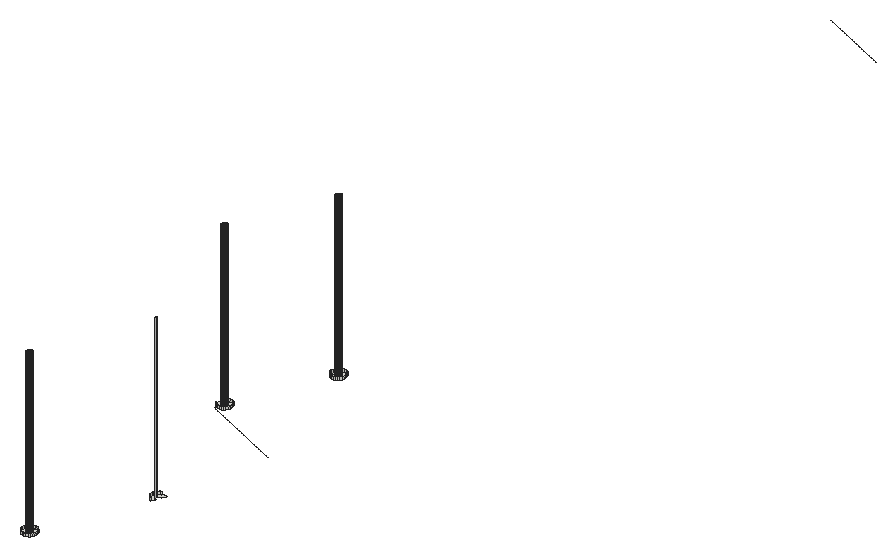
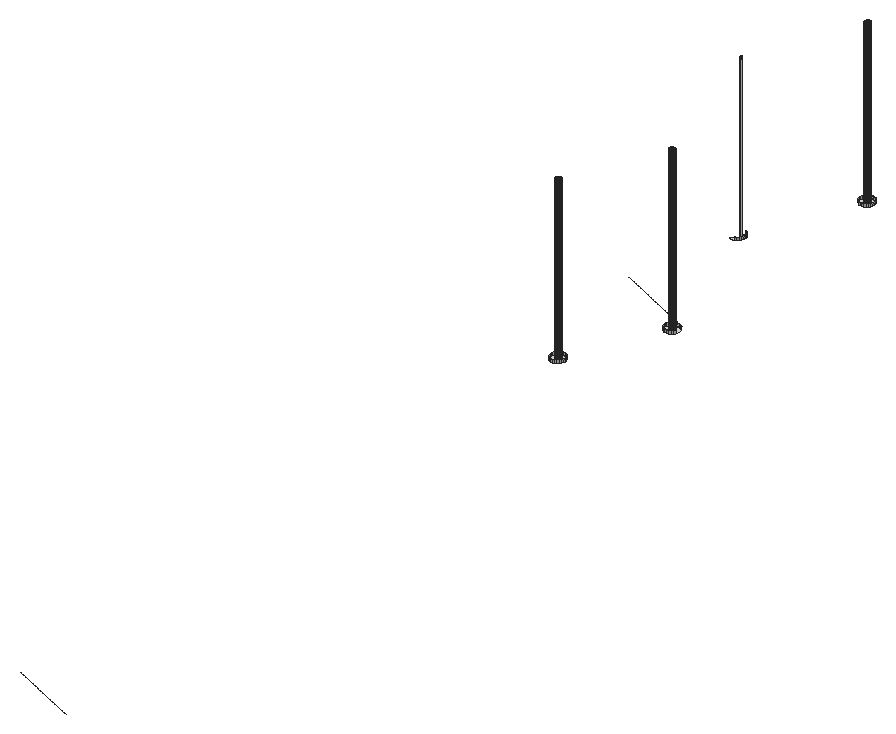
# SketchUp Ruby script. Lengths in inches.
U = 1.inch
M = Sketchup.active_model
def pt(a) = Geom::Point3d.new(a.map { |v| v * U })
def face(e, loops, mat)
  f = e.add_face(loops[0].map { |a| pt(a) })
  loops[1..].each { |l| e.add_face(l.map { |a| pt(a) }).erase! }
  f.material = f.back_material = mat if mat
  f
end
# faces: each face lists its corners as indices into pts; further lists are holes
def faces(e, pts, list, mat = nil) = list.each { |f| face(e, (f[0].is_a?(Array) ? f : [f]).map { |l| l.map { |i| pts[i] } }, mat) }
# xy, xz, yz: faces in a plane at the given z, y or x. An outline is a flat list of corners, or four numbers for a rectangle; further outlines are holes
def ring(l) = l.size == 4 ? [[l[0], l[1]], [l[2], l[1]], [l[2], l[3]], [l[0], l[3]]] : l.each_slice(2).to_a
def flat(e, list, mat, &to3) = list.each { |f| face(e, (f[0].is_a?(Array) ? f : [f]).map { |l| ring(l).map { |u, v| to3.(u, v) } }, mat) }
def xy(e, z, list, mat = nil) = flat(e, list, mat) { |x, y| [x, y, z] }
def xz(e, y, list, mat = nil) = flat(e, list, mat) { |x, z| [x, y, z] }
def yz(e, x, list, mat = nil) = flat(e, list, mat) { |y, z| [x, y, z] }
def lines(e, pts, list) = list.each { |a, b| e.add_line(pt(pts[a]), pt(pts[b])) }
# prism: a flat outline (further loops are holes) pulled along v
def prism(e, loops, v, mat = nil)
  f = face(e, loops, mat); d = Geom::Vector3d.new(v.map { |x| x * U })
  f.pushpull(f.normal.samedirection?(d) ? d.length : -d.length)
end
def box(e, o, s, mat = nil) = prism(e, [[o, [o[0] + s[0], o[1], o[2]], [o[0] + s[0], o[1] + s[1], o[2]], [o[0], o[1] + s[1], o[2]]]], [0, 0, s[2]], mat)
def at(x, y, z, deg = 0) = Geom::Transformation.translation(pt([x, y, z])) * Geom::Transformation.rotation(ORIGIN, Z_AXIS, deg.degrees)
def axes(o, x, y, z) = Geom::Transformation.new([*x, 0, *y, 0, *z, 0, *pt(o).to_a, 1])
def part(name) = M.definitions.add(name)
# library, detail: a bought-in or finely detailed component or shape, given as its bounding box
def library(name, o, s) = part(name).tap { |d| box(d.entities, o, s) }
def detail(e, o, s) = box(e.add_group.entities, o, s)
def put(e, d, t, mat = nil) = e.add_instance(d, t).tap { |i| i.material = mat if mat }
def group(e, t, mat = nil) = e.add_group.tap { |g| g.transformation = t; g.material = mat if mat }.entities
root = M.entities
M.materials.add("[Color_000]").color = [255, 255, 255]
xy(root,321.27,[[[963.53,810.32,963.9375,810.4,964.3,810.59,964.61,810.86,964.84,811.2,964.97,811.59,964.99,812,964.91,812.4,964.73,812.77,964.45,813.08,964.11,813.31,964.05,813.33,963.72,813.4375,963.31,813.46,962.91,813.38,962.54,813.19,962.23,812.92,962.01,812.58,961.875,812.1875,961.85,811.78,961.93,811.375,962.12,811.01,962.39,810.7,962.73,810.47,962.8,810.45,963.125,810.34],[963.47,811.26,963.3,811.27,963.17,811.3125,963.15,811.32,963.01,811.41,962.9,811.54,962.83,811.68,962.79,811.84,962.8,812.01,962.86,812.16,962.95,812.3,963.07,812.41,963.22,812.48,963.375,812.52,963.54,812.51,963.67,812.46,963.7,812.46,963.83,812.37,963.94,812.24,964.02,812.1,964.05,811.93,964.04,811.77,963.99,811.61,963.9,811.48,963.77,811.37,963.63,811.29]],[962.8,810.45,963.17,811.3125,963.15,811.32,963.01,811.41,962.9,811.54,962.83,811.68,962.79,811.84,962.8,812.01,962.86,812.16,962.95,812.3,963.07,812.41,963.22,812.48,963.375,812.52,963.54,812.51,963.67,812.46,964.05,813.33,963.72,813.4375,963.31,813.46,962.91,813.38,962.54,813.19,962.23,812.92,962.01,812.58,961.875,812.1875,961.85,811.78,961.93,811.375,962.12,811.01,962.39,810.7,962.73,810.47],[963.17,811.3125,963.67,812.46,963.54,812.51,963.375,812.52,963.22,812.48,963.07,812.41,962.95,812.3,962.86,812.16,962.8,812.01,962.79,811.84,962.83,811.68,962.9,811.54,963.01,811.41,963.15,811.32],[972.96,833.79,973.34,834.66,973.3125,834.66,973.18,834.75,973.07,834.88,972.99,835.02,972.96,835.1875,972.97,835.35,973.02,835.51,973.11,835.64,973.23,835.75,973.38,835.83,973.54,835.86,973.71,835.85,973.84,835.81,974.21,836.67,973.89,836.78,973.48,836.8,973.07,836.72,972.7,836.53,972.4,836.26,972.17,835.92,972.04,835.53,972.02,835.12,972.1,834.72,972.28,834.35,972.56,834.04,972.9,833.8125],[[961.92,866.71,962.32,866.79,962.6875,866.97,962.99,867.25,963.22,867.59,963.35,867.98,963.375,868.39,963.29,868.79,963.11,869.16,962.83,869.47,962.49,869.69,962.43,869.72,962.1,869.82,961.69,869.85,961.29,869.77,960.92,869.58,960.61,869.31,960.39,868.97,960.26,868.58,960.23,868.17,960.32,867.76,960.5,867.4,960.77,867.09,961.12,866.86,961.51,866.73],[961.85,867.65,961.68,867.66,961.55,867.7,961.53,867.71,961.39,867.8,961.28,867.93,961.21,868.07,961.18,868.23,961.18,868.4,961.24,868.55,961.33,868.69,961.45,868.8,961.6,868.875,961.76,868.91,961.92,868.9,962.05,868.85,962.08,868.84,962.22,868.75,962.32,868.63,962.4,868.48,962.43,868.32,962.42,868.16,962.37,868,962.28,867.87,962.16,867.76,962.01,867.68]],
  [961.18,866.84,961.55,867.7,961.53,867.71,961.39,867.8,961.28,867.93,961.21,868.07,961.18,868.23,961.18,868.4,961.24,868.55,961.33,868.69,961.45,868.8,961.6,868.875,961.76,868.91,961.92,868.9,962.05,868.85,962.43,869.72,962.1,869.82,961.69,869.85,961.29,869.77,960.92,869.58,960.61,869.31,960.39,868.97,960.26,868.58,960.23,868.17,960.32,867.76,960.5,867.4,960.77,867.09,961.12,866.86],[961.55,867.7,962.05,868.85,961.92,868.9,961.76,868.91,961.6,868.875,961.45,868.8,961.33,868.69,961.24,868.55,961.18,868.4,961.18,868.23,961.21,868.07,961.28,867.93,961.39,867.8,961.53,867.71],[[970.875,887.27,971.28,887.36,971.64,887.54,971.95,887.8125,972.18,888.16,972.31,888.55,972.33,888.96,972.25,889.36,972.06,889.73,971.79,890.04,971.45,890.26,971.06,890.39,970.65,890.42,970.25,890.33,969.88,890.15,969.57,889.875,969.34,889.53,969.21,889.14,969.19,888.73,969.27,888.33,969.46,887.96,969.73,887.65,970.07,887.43,970.46,887.3],[970.81,888.22,970.64,888.23,970.51,888.27,970.49,888.28,970.35,888.37,970.24,888.49,970.17,888.64,970.13,888.8,970.14,888.96,970.19,889.12,970.28,889.26,970.41,889.37,970.55,889.44,970.72,889.47,970.88,889.46,971.01,889.42,971.04,889.41,971.17,889.32,971.28,889.2,971.36,889.05,971.39,888.89,971.38,888.73,971.33,888.57,971.24,888.43,971.11,888.32,970.97,888.25]],[970.13,887.41,970.51,888.27,970.49,888.28,970.35,888.37,970.24,888.49,970.17,888.64,970.13,888.8,970.14,888.96,970.19,889.12,970.28,889.26,970.41,889.37,970.55,889.44,970.72,889.47,970.88,889.46,971.01,889.42,971.39,890.28,971.06,890.39,970.65,890.42,970.25,890.33,969.88,890.15,969.57,889.875,969.34,889.53,969.21,889.14,969.19,888.73,969.27,888.33,969.46,887.96,969.73,887.65,970.07,887.43],[970.51,888.27,971.01,889.42,970.88,889.46,970.72,889.47,970.55,889.44,970.41,889.37,970.28,889.26,970.19,889.12,970.14,888.96,970.13,888.8,970.17,888.64,970.24,888.49,970.35,888.37,970.49,888.28]])
xy(root,321.27,[[963.47,811.26,963.63,811.29,963.77,811.37,963.9,811.48,963.99,811.61,964.04,811.77,964.05,811.93,964.02,812.1,963.94,812.24,963.83,812.37,963.7,812.46,963.67,812.46,963.17,811.3125,963.3,811.27],[961.85,867.65,962.01,867.68,962.16,867.76,962.28,867.87,962.37,868,962.42,868.16,962.43,868.32,962.4,868.48,962.32,868.63,962.22,868.75,962.08,868.84,962.05,868.85,961.55,867.7,961.68,867.66],[970.81,888.22,970.97,888.25,971.11,888.32,971.24,888.43,971.33,888.57,971.38,888.73,971.39,888.89,971.36,889.05,971.28,889.2,971.17,889.32,971.04,889.41,971.01,889.42,970.51,888.27,970.64,888.23]],"[Color_000]")
yz(root,961.18,[[868.23,321.27,868.4,357.27]],"[Color_000]")
p = [[962.73,810.47,321.27],[962.8,810.45,321.27],[963.125,810.34,321.27],[963.125,810.34,321.86],[962.73,810.47,321.86],[963.53,810.32,321.27],
  [963.53,810.32,321.86],[963.9375,810.4,321.27],[963.9375,810.4,321.86],[964.3,810.59,321.27],[964.3,810.59,321.86],[962.39,810.7,321.27],
  [962.39,810.7,321.86],[964.61,810.86,321.27],[964.61,810.86,321.86],[962.12,811.01,321.27],[962.12,811.01,321.86],[964.84,811.2,321.27],
  [964.84,811.2,321.86],[961.93,811.375,321.27],[961.93,811.375,321.86],[964.97,811.59,321.27],[964.97,811.59,321.86],[963.01,811.41,321.27],
  [963.15,811.32,321.27],[963.15,811.32,357.27],[963.01,811.41,357.27],[963.17,811.3125,321.27],[963.3,811.27,321.27],[963.3,811.27,357.27],
  [963.47,811.26,321.27],[963.47,811.26,357.27],[963.63,811.29,321.27],[963.63,811.29,357.27],[963.77,811.37,321.27],[963.77,811.37,357.27],
  [961.85,811.78,321.27],[961.85,811.78,321.86],[962.9,811.54,321.27],[962.9,811.54,357.27],[963.9,811.48,321.27],[963.9,811.48,357.27],
  [962.83,811.68,321.27],[962.83,811.68,357.27],[963.99,811.61,321.27],[963.99,811.61,357.27],[964.04,811.77,321.27],[964.04,811.77,357.27],
  [964.99,812,321.27],[964.99,812,321.86],[962.79,811.84,321.27],[962.79,811.84,357.27],[961.875,812.1875,321.27],[961.875,812.1875,321.86],
  [962.8,812.01,321.27],[962.8,812.01,357.27],[964.05,811.93,321.27],[964.05,811.93,357.27],[964.02,812.1,321.27],[964.02,812.1,357.27],
  [962.86,812.16,321.27],[962.86,812.16,357.27],[964.91,812.4,321.27],[964.91,812.4,321.86],[963.94,812.24,321.27],[963.94,812.24,357.27],
  [962.01,812.58,321.27],[962.01,812.58,321.86],[962.95,812.3,321.27],[962.95,812.3,357.27],[963.83,812.37,321.27],[963.83,812.37,357.27],
  [963.07,812.41,321.27],[963.07,812.41,357.27],[963.22,812.48,321.27],[963.22,812.48,357.27],[963.7,812.46,321.27],[963.7,812.46,357.27],
  [964.73,812.77,321.27],[964.73,812.77,321.86],[963.375,812.52,321.27],[963.375,812.52,357.27],[963.54,812.51,321.27],[963.54,812.51,357.27],
  [963.67,812.46,321.27],[962.23,812.92,321.27],[962.23,812.92,321.86],[964.45,813.08,321.27],[964.45,813.08,321.86],[962.54,813.19,321.27],
  [962.54,813.19,321.86],[964.11,813.31,321.27],[964.11,813.31,321.86],[962.91,813.38,321.27],[962.91,813.38,321.86],[964.05,813.33,321.27],
  [963.72,813.4375,321.27],[963.72,813.4375,321.86],[963.31,813.46,321.27],[963.31,813.46,321.86],[972.56,834.04,321.27],[972.9,833.8125,321.27],
  [972.9,833.8125,321.86],[972.56,834.04,321.86],[972.28,834.35,321.27],[972.28,834.35,321.86],[972.1,834.72,321.27],[972.1,834.72,321.86],
  [972.02,835.12,321.27],[972.02,835.12,321.86],[972.99,835.02,321.27],[973.07,834.88,321.27],[973.07,834.88,357.27],[972.99,835.02,357.27],
  [972.96,835.1875,321.27],[972.96,835.1875,357.27],[972.04,835.53,321.27],[972.04,835.53,321.86],[972.97,835.35,321.27],[972.97,835.35,357.27],
  [973.02,835.51,321.27],[973.02,835.51,357.27],[972.17,835.92,321.27],[972.17,835.92,321.86],[972.4,836.26,321.27],[972.4,836.26,321.86],
  [972.7,836.53,321.27],[972.7,836.53,321.86],[973.07,836.72,321.27],[973.07,836.72,321.86],[961.12,866.86,321.27],[961.18,866.84,321.27],
  [961.51,866.73,321.27],[961.51,866.73,321.86],[961.12,866.86,321.86],[961.92,866.71,321.27],[961.92,866.71,321.86],[962.32,866.79,321.27],
  [962.32,866.79,321.86],[962.6875,866.97,321.27],[962.6875,866.97,321.86],[960.77,867.09,321.27],[960.77,867.09,321.86],[962.99,867.25,321.27],
  [962.99,867.25,321.86],[960.5,867.4,321.27],[960.5,867.4,321.86],[963.22,867.59,321.27],[963.22,867.59,321.86],[961.68,867.66,321.27],
  [961.85,867.65,321.27],[961.85,867.65,357.27],[961.68,867.66,357.27],[962.01,867.68,321.27],[962.01,867.68,357.27],[963.35,867.98,321.27],
  [963.35,867.98,321.86],[961.39,867.8,321.27],[961.53,867.71,321.27],[961.53,867.71,357.27],[961.39,867.8,357.27],[961.55,867.7,321.27],
  [962.16,867.76,321.27],[962.16,867.76,357.27],[961.28,867.93,321.27],[961.28,867.93,357.27],[962.28,867.87,321.27],[962.28,867.87,357.27],
  [961.21,868.07,321.27],[961.21,868.07,357.27],[962.37,868,321.27],[962.37,868,357.27],[962.42,868.16,321.27],[962.42,868.16,357.27],
  [963.375,868.39,321.27],[963.375,868.39,321.86],[961.18,868.23,321.27],[961.18,868.23,357.27],[962.43,868.32,321.27],[962.43,868.32,357.27],
  [962.4,868.48,321.27],[962.4,868.48,357.27],[961.24,868.55,321.27],[961.18,868.4,321.27],[961.18,868.4,357.27],[961.24,868.55,357.27],
  [963.29,868.79,321.27],[963.29,868.79,321.86],[962.32,868.63,321.27],[962.32,868.63,357.27],[961.33,868.69,321.27],[961.33,868.69,357.27],
  [962.22,868.75,321.27],[962.22,868.75,357.27],[961.45,868.8,321.27],[961.45,868.8,357.27],[961.6,868.875,321.27],[961.6,868.875,357.27],
  [962.08,868.84,321.27],[962.05,868.85,321.27],[961.92,868.9,321.27],[961.92,868.9,357.27],[962.08,868.84,357.27],[963.11,869.16,321.27],
  [963.11,869.16,321.86],[961.76,868.91,321.27],[961.76,868.91,357.27],[960.61,869.31,321.27],[960.39,868.97,321.27],[960.39,868.97,321.86],
  [960.61,869.31,321.86],[962.83,869.47,321.27],[962.83,869.47,321.86],[960.92,869.58,321.27],[960.92,869.58,321.86],[962.49,869.69,321.27],
  [962.49,869.69,321.86],[961.29,869.77,321.27],[961.29,869.77,321.86],[962.43,869.72,321.27],[962.1,869.82,321.27],[962.1,869.82,321.86],
  [961.69,869.85,321.27],[961.69,869.85,321.86],[970.07,887.43,321.27],[970.13,887.41,321.27],[970.46,887.3,321.27],[970.46,887.3,321.86],
  [970.07,887.43,321.86],[970.875,887.27,321.27],[970.875,887.27,321.86],[971.28,887.36,321.27],[971.28,887.36,321.86],[969.73,887.65,321.27],
  [969.73,887.65,321.86],[971.64,887.54,321.27],[971.64,887.54,321.86],[971.95,887.8125,321.27],[971.95,887.8125,321.86],[969.46,887.96,321.27],
  [969.46,887.96,321.86],[972.18,888.16,321.27],[972.18,888.16,321.86],[969.27,888.33,321.27],[969.27,888.33,321.86],[970.49,888.28,321.27],
  [970.51,888.27,321.27],[970.64,888.23,321.27],[970.64,888.23,357.27],[970.49,888.28,357.27],[970.81,888.22,321.27],[970.81,888.22,357.27],
  [970.97,888.25,321.27],[970.97,888.25,357.27],[971.11,888.32,321.27],[971.11,888.32,357.27],[972.31,888.55,321.27],[972.31,888.55,321.86],
  [969.19,888.73,321.27],[969.19,888.73,321.86],[970.35,888.37,321.27],[970.35,888.37,357.27],[971.24,888.43,321.27],[971.24,888.43,357.27],
  [970.24,888.49,321.27],[970.24,888.49,357.27],[971.33,888.57,321.27],[971.33,888.57,357.27],[970.17,888.64,321.27],[970.17,888.64,357.27],
  [972.33,888.96,321.27],[972.33,888.96,321.86],[970.13,888.8,321.27],[970.13,888.8,357.27],[971.38,888.73,321.27],[971.38,888.73,357.27],
  [969.21,889.14,321.27],[969.21,889.14,321.86],[971.39,888.89,321.27],[971.39,888.89,357.27],[970.14,888.96,321.27],[970.14,888.96,357.27],
  [971.36,889.05,321.27],[971.36,889.05,357.27],[970.19,889.12,321.27],[970.19,889.12,357.27],[972.25,889.36,321.27],[972.25,889.36,321.86],
  [969.34,889.53,321.27],[969.34,889.53,321.86],[970.28,889.26,321.27],[970.28,889.26,357.27],[971.28,889.2,321.27],[971.28,889.2,357.27],
  [971.17,889.32,321.27],[971.17,889.32,357.27],[970.41,889.37,321.27],[970.41,889.37,357.27],[971.04,889.41,321.27],[971.04,889.41,357.27],
  [970.55,889.44,321.27],[970.55,889.44,357.27],[970.72,889.47,321.27],[970.72,889.47,357.27],[971.01,889.42,321.27],[970.88,889.46,321.27],
  [970.88,889.46,357.27],[972.06,889.73,321.27],[972.06,889.73,321.86],[969.57,889.875,321.27],[969.57,889.875,321.86],[971.79,890.04,321.27],
  [971.79,890.04,321.86],[969.88,890.15,321.27],[969.88,890.15,321.86],[971.45,890.26,321.27],[971.45,890.26,321.86],[970.25,890.33,321.27],
  [970.25,890.33,321.86],[970.65,890.42,321.27],[970.65,890.42,321.86],[971.39,890.28,321.27],[971.06,890.39,321.27],[971.06,890.39,321.86],
  [961,866.44,321.27],[979.33,858.46,321.27],[974.34,1034.0625,321.27],[958.76,1040.85,321.27]]
faces(root,p,[[0,1,2,3,4],[2,5,6,3],[5,7,8,6],[7,9,10,8],[11,0,4,12],[9,13,14,10],[15,11,12,16],[13,17,18,14],
  [19,15,16,20],[17,21,22,18],[36,19,20,37],[21,48,49,22],[52,36,37,53],[48,62,63,49],[66,52,53,67],[62,78,79,63],
  [85,66,67,86],[78,87,88,79],[89,85,86,90],[87,91,92,88],[93,89,90,94],[91,95,96,97,92],[98,93,94,99],[96,98,99,97],
  [100,101,102,103],[104,100,103,105],[106,104,105,107],[108,106,107,109],[116,108,109,117],[122,116,117,123],[124,122,123,125],[126,124,125,127],
  [128,126,127,129],[130,131,132,133,134],[132,135,136,133],[135,137,138,136],[137,139,140,138],[141,130,134,142],[139,143,144,140],[145,141,142,146],
  [143,147,148,144],[147,155,156,148],[155,174,175,156],[174,186,187,175],[186,203,204,187],[207,208,209,210],[203,211,212,204],[213,207,210,214],
  [211,215,216,212],[217,213,214,218],[215,219,220,221,216],[222,217,218,223],[220,222,223,221],[224,225,226,227,228],[226,229,230,227],[229,231,232,230],
  [233,224,228,234],[231,235,236,232],[235,237,238,236],[239,233,234,240],[237,241,242,238],[243,239,240,244],[241,256,257,242],[258,243,244,259],
  [256,270,271,257],[276,258,259,277],[270,286,287,271],[288,276,277,289],[286,307,308,287],[309,288,289,310],[307,311,312,308],[313,309,310,314],
  [311,315,316,312],[317,313,314,318],[319,317,318,320],[315,321,322,323,316],[322,319,320,323]])
faces(root,p,[[23,24,25,26],[24,27,28,29,25],[28,30,31,29],[30,32,33,31],[32,34,35,33],[38,23,26,39],[34,40,41,35],[42,38,39,43],
  [40,44,45,41],[44,46,47,45],[50,42,43,51],[54,50,51,55],[46,56,57,47],[56,58,59,57],[60,54,55,61],[58,64,65,59],
  [68,60,61,69],[64,70,71,65],[72,68,69,73],[74,72,73,75],[70,76,77,71],[80,74,75,81],[82,80,81,83],[76,84,82,83,77],
  [110,111,112,113],[114,110,113,115],[118,114,115,119],[120,118,119,121],[149,150,151,152],[150,153,154,151],[157,158,159,160],[158,161,149,152,159],
  [153,162,163,154],[164,157,160,165],[162,166,167,163],[168,164,165,169],[166,170,171,167],[170,172,173,171],[176,168,169,177],[172,178,179,173],
  [178,180,181,179],[182,183,184,185],[180,188,189,181],[190,182,185,191],[188,192,193,189],[194,190,191,195],[196,194,195,197],[198,199,200,201,202],
  [192,198,202,193],[205,196,197,206],[200,205,206,201],[245,246,247,248,249],[247,250,251,248],[250,252,253,251],[252,254,255,253],[260,245,249,261],
  [254,262,263,255],[264,260,261,265],[262,266,267,263],[268,264,265,269],[272,268,269,273],[266,274,275,267],[274,278,279,275],[280,272,273,281],
  [278,282,283,279],[284,280,281,285],[290,284,285,291],[282,292,293,283],[292,294,295,293],[296,290,291,297],[294,298,299,295],[300,296,297,301],
  [302,300,301,303],[298,304,305,306,299],[305,302,303,306]],"[Color_000]")
lines(root,p,[[324,131],[325,324],[326,327]])
